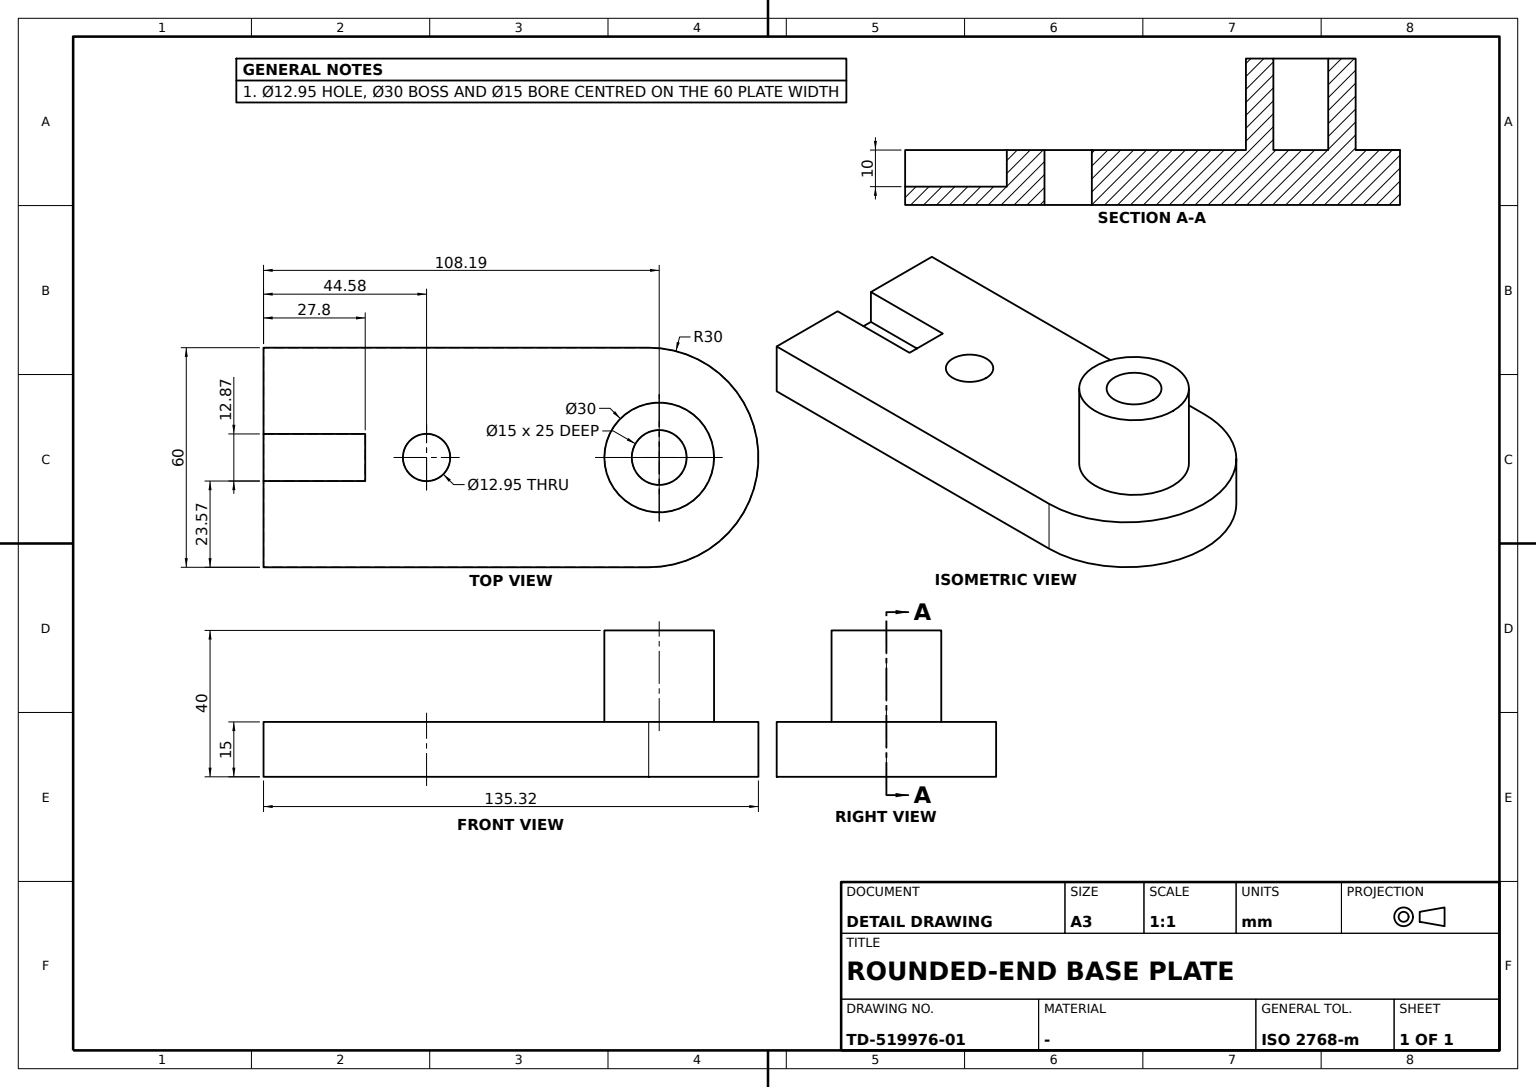
ISO-10303-21;
HEADER;
FILE_DESCRIPTION((''),'2;1');
FILE_NAME('','',(''),(''),'','','');
FILE_SCHEMA(('AUTOMOTIVE_DESIGN'));
ENDSEC;
DATA;
#1=APPLICATION_CONTEXT('');
#2=PRODUCT_CONTEXT('',#1,'mechanical');
#3=PRODUCT('','','',(#2));
#4=PRODUCT_DEFINITION_FORMATION('','',#3);
#5=PRODUCT_DEFINITION_CONTEXT('',#1,'design');
#6=PRODUCT_DEFINITION('','',#4,#5);
#7=PRODUCT_DEFINITION_SHAPE('','',#6);
#8=(LENGTH_UNIT()NAMED_UNIT(*)SI_UNIT(.MILLI.,.METRE.));
#9=(NAMED_UNIT(*)PLANE_ANGLE_UNIT()SI_UNIT($,.RADIAN.));
#10=(NAMED_UNIT(*)SI_UNIT($,.STERADIAN.)SOLID_ANGLE_UNIT());
#11=UNCERTAINTY_MEASURE_WITH_UNIT(LENGTH_MEASURE(0.005),#8,'distance_accuracy_value','');
#12=(GEOMETRIC_REPRESENTATION_CONTEXT(3)GLOBAL_UNCERTAINTY_ASSIGNED_CONTEXT((#11))GLOBAL_UNIT_ASSIGNED_CONTEXT((#8,#9,#10))REPRESENTATION_CONTEXT('',''));
#13=CARTESIAN_POINT('',(-37.355505,6.43284,15.));
#14=VERTEX_POINT('',#13);
#15=CARTESIAN_POINT('',(-37.355505,-6.43284,15.));
#16=VERTEX_POINT('',#15);
#17=DIRECTION('',(0.,-1.,0.));
#18=VECTOR('',#17,1000.);
#19=LINE('',#13,#18);
#20=EDGE_CURVE('',#14,#16,#19,.T.);
#21=ORIENTED_EDGE('',*,*,#20,.F.);
#22=CARTESIAN_POINT('',(-37.355505,6.43284,5.));
#23=VERTEX_POINT('',#22);
#24=DIRECTION('',(0.,0.,-1.));
#25=VECTOR('',#24,1000.);
#26=LINE('',#13,#25);
#27=EDGE_CURVE('',#14,#23,#26,.T.);
#28=ORIENTED_EDGE('',*,*,#27,.T.);
#29=CARTESIAN_POINT('',(-37.355505,-6.43284,5.));
#30=VERTEX_POINT('',#29);
#31=LINE('',#22,#18);
#32=EDGE_CURVE('',#23,#30,#31,.T.);
#33=ORIENTED_EDGE('',*,*,#32,.T.);
#34=LINE('',#15,#25);
#35=EDGE_CURVE('',#16,#30,#34,.T.);
#36=ORIENTED_EDGE('',*,*,#35,.F.);
#37=EDGE_LOOP('',(#21,#28,#33,#36));
#38=FACE_BOUND('',#37,.T.);
#39=DIRECTION('',(1.,0.,0.));
#40=AXIS2_PLACEMENT_3D('',#13,#39,#17);
#41=PLANE('',#40);
#42=ADVANCED_FACE('',(#38),#41,.F.);
#43=CARTESIAN_POINT('',(-65.157942,6.43284,5.));
#44=VERTEX_POINT('',#43);
#45=CARTESIAN_POINT('',(-92.577634,6.43284,5.));
#46=VECTOR('',#39,1000.);
#47=LINE('',#45,#46);
#48=EDGE_CURVE('',#44,#23,#47,.T.);
#49=ORIENTED_EDGE('',*,*,#48,.T.);
#50=ORIENTED_EDGE('',*,*,#27,.F.);
#51=CARTESIAN_POINT('',(-65.157942,6.43284,15.));
#52=VERTEX_POINT('',#51);
#53=CARTESIAN_POINT('',(-92.577634,6.43284,15.));
#54=LINE('',#53,#46);
#55=EDGE_CURVE('',#52,#14,#54,.T.);
#56=ORIENTED_EDGE('',*,*,#55,.F.);
#57=LINE('',#51,#25);
#58=EDGE_CURVE('',#52,#44,#57,.T.);
#59=ORIENTED_EDGE('',*,*,#58,.T.);
#60=EDGE_LOOP('',(#49,#50,#56,#59));
#61=FACE_BOUND('',#60,.T.);
#62=DIRECTION('',(0.,1.,0.));
#63=AXIS2_PLACEMENT_3D('',#53,#62,#39);
#64=PLANE('',#63);
#65=ADVANCED_FACE('',(#61),#64,.F.);
#66=CARTESIAN_POINT('',(40.157942,-30.,0.));
#67=VERTEX_POINT('',#66);
#68=CARTESIAN_POINT('',(-65.157942,-30.,0.));
#69=VERTEX_POINT('',#68);
#70=CARTESIAN_POINT('',(0.,-30.,0.));
#71=DIRECTION('',(-1.,0.,0.));
#72=VECTOR('',#71,1000.);
#73=LINE('',#70,#72);
#74=EDGE_CURVE('',#67,#69,#73,.T.);
#75=ORIENTED_EDGE('',*,*,#74,.T.);
#76=CARTESIAN_POINT('',(-65.157942,30.,0.));
#77=VERTEX_POINT('',#76);
#78=CARTESIAN_POINT('',(-65.157942,0.,0.));
#79=VECTOR('',#62,1000.);
#80=LINE('',#78,#79);
#81=EDGE_CURVE('',#69,#77,#80,.T.);
#82=ORIENTED_EDGE('',*,*,#81,.T.);
#83=CARTESIAN_POINT('',(40.157942,30.,0.));
#84=VERTEX_POINT('',#83);
#85=CARTESIAN_POINT('',(0.,30.,0.));
#86=LINE('',#85,#46);
#87=EDGE_CURVE('',#77,#84,#86,.T.);
#88=ORIENTED_EDGE('',*,*,#87,.T.);
#89=CARTESIAN_POINT('',(40.157942,0.,0.));
#90=DIRECTION('',(0.,0.,1.));
#91=AXIS2_PLACEMENT_3D('',#89,#90,#39);
#92=CIRCLE('',#91,30.);
#93=EDGE_CURVE('',#67,#84,#92,.T.);
#94=ORIENTED_EDGE('',*,*,#93,.F.);
#95=EDGE_LOOP('',(#75,#82,#88,#94));
#96=FACE_BOUND('',#95,.T.);
#97=CARTESIAN_POINT('',(-14.105343,0.,0.));
#98=VERTEX_POINT('',#97);
#99=CARTESIAN_POINT('',(-20.579161,0.,0.));
#100=AXIS2_PLACEMENT_3D('',#99,#90,#39);
#101=CIRCLE('',#100,6.473818);
#102=EDGE_CURVE('',#98,#98,#101,.T.);
#103=ORIENTED_EDGE('',*,*,#102,.T.);
#104=EDGE_LOOP('',(#103));
#105=FACE_BOUND('',#104,.T.);
#106=CARTESIAN_POINT('',(0.,0.,0.));
#107=AXIS2_PLACEMENT_3D('',#106,#90,#39);
#108=PLANE('',#107);
#109=ADVANCED_FACE('',(#96,#105),#108,.F.);
#110=CARTESIAN_POINT('',(50.531142,0.,40.));
#111=VERTEX_POINT('',#110);
#112=CARTESIAN_POINT('',(43.031142,0.,40.));
#113=AXIS2_PLACEMENT_3D('',#112,#90,#39);
#114=CIRCLE('',#113,7.5);
#115=EDGE_CURVE('',#111,#111,#114,.T.);
#116=ORIENTED_EDGE('',*,*,#115,.T.);
#117=EDGE_LOOP('',(#116));
#118=FACE_BOUND('',#117,.T.);
#119=CARTESIAN_POINT('',(50.531142,0.,15.));
#120=VERTEX_POINT('',#119);
#121=CARTESIAN_POINT('',(43.031142,0.,15.));
#122=AXIS2_PLACEMENT_3D('',#121,#90,#39);
#123=CIRCLE('',#122,7.5);
#124=EDGE_CURVE('',#120,#120,#123,.T.);
#125=ORIENTED_EDGE('',*,*,#124,.F.);
#126=EDGE_LOOP('',(#125));
#127=FACE_BOUND('',#126,.T.);
#128=CARTESIAN_POINT('',(43.031142,0.,27.5));
#129=AXIS2_PLACEMENT_3D('',#128,#90,#39);
#130=CYLINDRICAL_SURFACE('',#129,7.5);
#131=ADVANCED_FACE('',(#118,#127),#130,.F.);
#132=CARTESIAN_POINT('',(-14.105343,0.,15.));
#133=VERTEX_POINT('',#132);
#134=CARTESIAN_POINT('',(-20.579161,0.,15.));
#135=AXIS2_PLACEMENT_3D('',#134,#90,#39);
#136=CIRCLE('',#135,6.473818);
#137=EDGE_CURVE('',#133,#133,#136,.T.);
#138=ORIENTED_EDGE('',*,*,#137,.T.);
#139=EDGE_LOOP('',(#138));
#140=FACE_BOUND('',#139,.T.);
#141=ORIENTED_EDGE('',*,*,#102,.F.);
#142=EDGE_LOOP('',(#141));
#143=FACE_BOUND('',#142,.T.);
#144=CARTESIAN_POINT('',(-20.579161,0.,6.84));
#145=AXIS2_PLACEMENT_3D('',#144,#90,#39);
#146=CYLINDRICAL_SURFACE('',#145,6.473818);
#147=ADVANCED_FACE('',(#140,#143),#146,.F.);
#148=CARTESIAN_POINT('',(40.157942,-30.,15.));
#149=VERTEX_POINT('',#148);
#150=CARTESIAN_POINT('',(40.157942,30.,15.));
#151=VERTEX_POINT('',#150);
#152=CARTESIAN_POINT('',(40.157942,0.,15.));
#153=AXIS2_PLACEMENT_3D('',#152,#90,#39);
#154=CIRCLE('',#153,30.);
#155=EDGE_CURVE('',#149,#151,#154,.T.);
#156=ORIENTED_EDGE('',*,*,#155,.F.);
#157=CARTESIAN_POINT('',(40.157942,-30.,7.5));
#158=VECTOR('',#90,1000.);
#159=LINE('',#157,#158);
#160=EDGE_CURVE('',#67,#149,#159,.T.);
#161=ORIENTED_EDGE('',*,*,#160,.F.);
#162=ORIENTED_EDGE('',*,*,#93,.T.);
#163=CARTESIAN_POINT('',(40.157942,30.,7.5));
#164=LINE('',#163,#158);
#165=EDGE_CURVE('',#84,#151,#164,.T.);
#166=ORIENTED_EDGE('',*,*,#165,.T.);
#167=EDGE_LOOP('',(#156,#161,#162,#166));
#168=FACE_BOUND('',#167,.T.);
#169=CARTESIAN_POINT('',(40.157942,0.,7.5));
#170=AXIS2_PLACEMENT_3D('',#169,#90,#39);
#171=CYLINDRICAL_SURFACE('',#170,30.);
#172=ADVANCED_FACE('',(#168),#171,.T.);
#173=CARTESIAN_POINT('',(58.031142,0.,15.));
#174=VERTEX_POINT('',#173);
#175=CIRCLE('',#122,15.);
#176=EDGE_CURVE('',#174,#174,#175,.T.);
#177=ORIENTED_EDGE('',*,*,#176,.T.);
#178=EDGE_LOOP('',(#177));
#179=FACE_BOUND('',#178,.T.);
#180=CARTESIAN_POINT('',(58.031142,0.,40.));
#181=VERTEX_POINT('',#180);
#182=CIRCLE('',#113,15.);
#183=EDGE_CURVE('',#181,#181,#182,.T.);
#184=ORIENTED_EDGE('',*,*,#183,.F.);
#185=EDGE_LOOP('',(#184));
#186=FACE_BOUND('',#185,.T.);
#187=CYLINDRICAL_SURFACE('',#129,15.);
#188=ADVANCED_FACE('',(#179,#186),#187,.T.);
#189=ORIENTED_EDGE('',*,*,#32,.F.);
#190=ORIENTED_EDGE('',*,*,#48,.F.);
#191=CARTESIAN_POINT('',(-65.157942,-6.43284,5.));
#192=VERTEX_POINT('',#191);
#193=CARTESIAN_POINT('',(-65.157942,-30.,5.));
#194=LINE('',#193,#18);
#195=EDGE_CURVE('',#44,#192,#194,.T.);
#196=ORIENTED_EDGE('',*,*,#195,.T.);
#197=LINE('',#29,#72);
#198=EDGE_CURVE('',#30,#192,#197,.T.);
#199=ORIENTED_EDGE('',*,*,#198,.F.);
#200=EDGE_LOOP('',(#189,#190,#196,#199));
#201=FACE_BOUND('',#200,.T.);
#202=CARTESIAN_POINT('',(0.,0.,5.));
#203=AXIS2_PLACEMENT_3D('',#202,#90,#39);
#204=PLANE('',#203);
#205=ADVANCED_FACE('',(#201),#204,.T.);
#206=ORIENTED_EDGE('',*,*,#124,.T.);
#207=EDGE_LOOP('',(#206));
#208=FACE_BOUND('',#207,.T.);
#209=CARTESIAN_POINT('',(0.,0.,15.));
#210=AXIS2_PLACEMENT_3D('',#209,#90,#39);
#211=PLANE('',#210);
#212=ADVANCED_FACE('',(#208),#211,.T.);
#213=ORIENTED_EDGE('',*,*,#176,.F.);
#214=EDGE_LOOP('',(#213));
#215=FACE_BOUND('',#214,.T.);
#216=ORIENTED_EDGE('',*,*,#137,.F.);
#217=EDGE_LOOP('',(#216));
#218=FACE_BOUND('',#217,.T.);
#219=ORIENTED_EDGE('',*,*,#20,.T.);
#220=CARTESIAN_POINT('',(-65.157942,-6.43284,15.));
#221=VERTEX_POINT('',#220);
#222=LINE('',#15,#72);
#223=EDGE_CURVE('',#16,#221,#222,.T.);
#224=ORIENTED_EDGE('',*,*,#223,.T.);
#225=CARTESIAN_POINT('',(-65.157942,-30.,15.));
#226=VERTEX_POINT('',#225);
#227=CARTESIAN_POINT('',(-65.157942,0.,15.));
#228=LINE('',#227,#79);
#229=EDGE_CURVE('',#226,#221,#228,.T.);
#230=ORIENTED_EDGE('',*,*,#229,.F.);
#231=CARTESIAN_POINT('',(0.,-30.,15.));
#232=LINE('',#231,#72);
#233=EDGE_CURVE('',#149,#226,#232,.T.);
#234=ORIENTED_EDGE('',*,*,#233,.F.);
#235=ORIENTED_EDGE('',*,*,#155,.T.);
#236=CARTESIAN_POINT('',(-65.157942,30.,15.));
#237=VERTEX_POINT('',#236);
#238=CARTESIAN_POINT('',(0.,30.,15.));
#239=LINE('',#238,#46);
#240=EDGE_CURVE('',#237,#151,#239,.T.);
#241=ORIENTED_EDGE('',*,*,#240,.F.);
#242=EDGE_CURVE('',#52,#237,#228,.T.);
#243=ORIENTED_EDGE('',*,*,#242,.F.);
#244=ORIENTED_EDGE('',*,*,#55,.T.);
#245=EDGE_LOOP('',(#219,#224,#230,#234,#235,#241,#243,#244));
#246=FACE_BOUND('',#245,.T.);
#247=ADVANCED_FACE('',(#215,#218,#246),#211,.T.);
#248=ORIENTED_EDGE('',*,*,#115,.F.);
#249=EDGE_LOOP('',(#248));
#250=FACE_BOUND('',#249,.T.);
#251=ORIENTED_EDGE('',*,*,#183,.T.);
#252=EDGE_LOOP('',(#251));
#253=FACE_BOUND('',#252,.T.);
#254=CARTESIAN_POINT('',(0.,0.,40.));
#255=AXIS2_PLACEMENT_3D('',#254,#90,#39);
#256=PLANE('',#255);
#257=ADVANCED_FACE('',(#250,#253),#256,.T.);
#258=ORIENTED_EDGE('',*,*,#81,.F.);
#259=LINE('',#68,#158);
#260=EDGE_CURVE('',#69,#226,#259,.T.);
#261=ORIENTED_EDGE('',*,*,#260,.T.);
#262=ORIENTED_EDGE('',*,*,#229,.T.);
#263=CARTESIAN_POINT('',(-65.157942,-6.43284,0.));
#264=LINE('',#263,#25);
#265=EDGE_CURVE('',#221,#192,#264,.T.);
#266=ORIENTED_EDGE('',*,*,#265,.T.);
#267=ORIENTED_EDGE('',*,*,#195,.F.);
#268=ORIENTED_EDGE('',*,*,#58,.F.);
#269=ORIENTED_EDGE('',*,*,#242,.T.);
#270=LINE('',#76,#158);
#271=EDGE_CURVE('',#77,#237,#270,.T.);
#272=ORIENTED_EDGE('',*,*,#271,.F.);
#273=EDGE_LOOP('',(#258,#261,#262,#266,#267,#268,#269,#272));
#274=FACE_BOUND('',#273,.T.);
#275=AXIS2_PLACEMENT_3D('',#68,#39,#62);
#276=PLANE('',#275);
#277=ADVANCED_FACE('',(#274),#276,.F.);
#278=ORIENTED_EDGE('',*,*,#260,.F.);
#279=ORIENTED_EDGE('',*,*,#74,.F.);
#280=ORIENTED_EDGE('',*,*,#160,.T.);
#281=ORIENTED_EDGE('',*,*,#233,.T.);
#282=EDGE_LOOP('',(#278,#279,#280,#281));
#283=FACE_BOUND('',#282,.T.);
#284=AXIS2_PLACEMENT_3D('',#66,#62,#71);
#285=PLANE('',#284);
#286=ADVANCED_FACE('',(#283),#285,.F.);
#287=ORIENTED_EDGE('',*,*,#240,.T.);
#288=ORIENTED_EDGE('',*,*,#165,.F.);
#289=ORIENTED_EDGE('',*,*,#87,.F.);
#290=ORIENTED_EDGE('',*,*,#271,.T.);
#291=EDGE_LOOP('',(#287,#288,#289,#290));
#292=FACE_BOUND('',#291,.T.);
#293=AXIS2_PLACEMENT_3D('',#76,#17,#39);
#294=PLANE('',#293);
#295=ADVANCED_FACE('',(#292),#294,.F.);
#296=ORIENTED_EDGE('',*,*,#265,.F.);
#297=ORIENTED_EDGE('',*,*,#223,.F.);
#298=ORIENTED_EDGE('',*,*,#35,.T.);
#299=ORIENTED_EDGE('',*,*,#198,.T.);
#300=EDGE_LOOP('',(#296,#297,#298,#299));
#301=FACE_BOUND('',#300,.T.);
#302=AXIS2_PLACEMENT_3D('',#15,#17,#71);
#303=PLANE('',#302);
#304=ADVANCED_FACE('',(#301),#303,.F.);
#305=CLOSED_SHELL('',(#42,#65,#109,#131,#147,#172,#188,#205,#212,#247,#257,#277,#286,#295,#304));
#306=MANIFOLD_SOLID_BREP('',#305);
#307=ADVANCED_BREP_SHAPE_REPRESENTATION('',(#306),#12);
#308=SHAPE_DEFINITION_REPRESENTATION(#7,#307);
ENDSEC;
END-ISO-10303-21;
